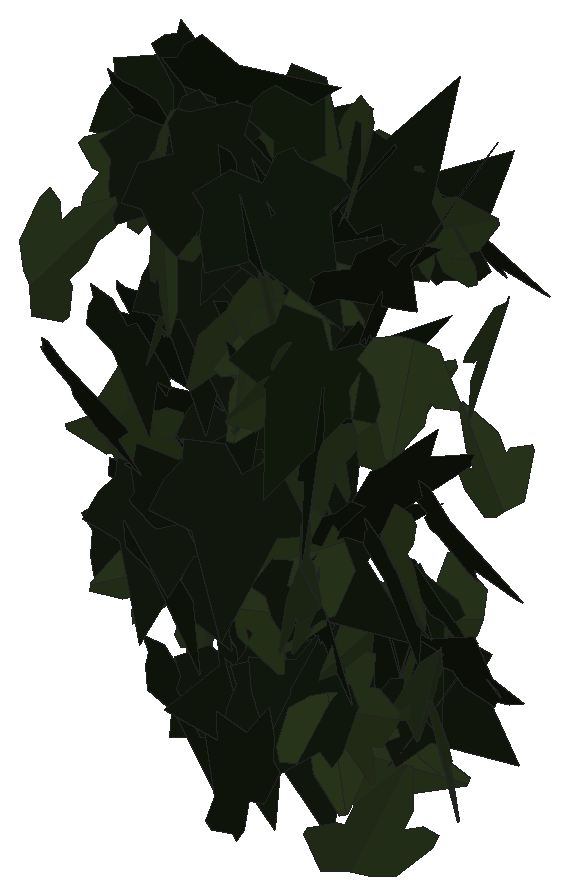
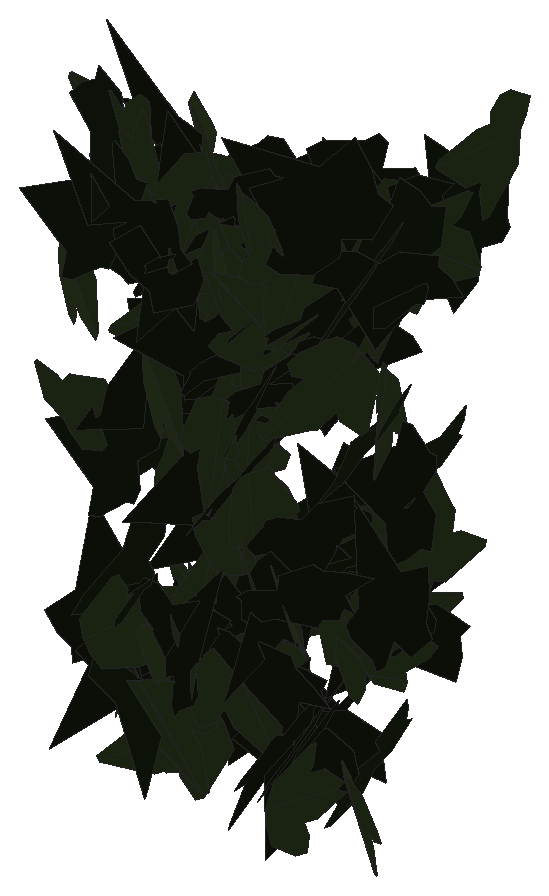
# SketchUp Ruby script. Lengths in inches.
U = 1.inch
M = Sketchup.active_model
def pt(a) = Geom::Point3d.new(a.map { |v| v * U })
def face(e, loops, mat)
  f = e.add_face(loops[0].map { |a| pt(a) })
  loops[1..].each { |l| e.add_face(l.map { |a| pt(a) }).erase! }
  f.material = f.back_material = mat if mat
  f
end
# faces: each face lists its corners as indices into pts; further lists are holes
def faces(e, pts, list, mat = nil) = list.each { |f| face(e, (f[0].is_a?(Array) ? f : [f]).map { |l| l.map { |i| pts[i] } }, mat) }
# xy, xz, yz: faces in a plane at the given z, y or x. An outline is a flat list of corners, or four numbers for a rectangle; further outlines are holes
def ring(l) = l.size == 4 ? [[l[0], l[1]], [l[2], l[1]], [l[2], l[3]], [l[0], l[3]]] : l.each_slice(2).to_a
def flat(e, list, mat, &to3) = list.each { |f| face(e, (f[0].is_a?(Array) ? f : [f]).map { |l| ring(l).map { |u, v| to3.(u, v) } }, mat) }
def xy(e, z, list, mat = nil) = flat(e, list, mat) { |x, y| [x, y, z] }
def xz(e, y, list, mat = nil) = flat(e, list, mat) { |x, z| [x, y, z] }
def yz(e, x, list, mat = nil) = flat(e, list, mat) { |y, z| [x, y, z] }
def lines(e, pts, list) = list.each { |a, b| e.add_line(pt(pts[a]), pt(pts[b])) }
# prism: a flat outline (further loops are holes) pulled along v
def prism(e, loops, v, mat = nil)
  f = face(e, loops, mat); d = Geom::Vector3d.new(v.map { |x| x * U })
  f.pushpull(f.normal.samedirection?(d) ? d.length : -d.length)
end
def box(e, o, s, mat = nil) = prism(e, [[o, [o[0] + s[0], o[1], o[2]], [o[0] + s[0], o[1] + s[1], o[2]], [o[0], o[1] + s[1], o[2]]]], [0, 0, s[2]], mat)
def at(x, y, z, deg = 0) = Geom::Transformation.translation(pt([x, y, z])) * Geom::Transformation.rotation(ORIGIN, Z_AXIS, deg.degrees)
def axes(o, x, y, z) = Geom::Transformation.new([*x, 0, *y, 0, *z, 0, *pt(o).to_a, 1])
def part(name) = M.definitions.add(name)
# library, detail: a bought-in or finely detailed component or shape, given as its bounding box
def library(name, o, s) = part(name).tap { |d| box(d.entities, o, s) }
def detail(e, o, s) = box(e.add_group.entities, o, s)
def put(e, d, t, mat = nil) = e.add_instance(d, t).tap { |i| i.material = mat if mat }
def group(e, t, mat = nil) = e.add_group.tap { |g| g.transformation = t; g.material = mat if mat }.entities
root = M.entities
M.materials.add("efeu1").color = [18, 25, 13]
M.materials.add("efeu2").color = [43, 57, 29]
c1 = part("ivyleaf_9")
p = [[1.54,2.16,1.25],[1.36,2.04,1.19],[-0.21,0.99,0.68],[-0.71,1.11,0.82],[-0.85,0.86,0.67],[-0.8,0.17,0.21],
  [-0.9,-0.01,0.1],[-0.67,-0.16,-0.02],[-0.08,-0.08,-0.05],[-0.03,-0.6,-0.4],[0.65,-0.88,-0.66],[0.83,-0.6,-0.49],
  [1.29,-0.42,-0.43],[1.8125,-0.07,-0.26],[1.21,0.44,0.15]]
faces(c1.entities,p,[[0,1,2,3,4,5,6,7,8,9,10,11,12,13,14]],"efeu1")
c2 = part("ivyleaf_10")
p = [[0,0.5,-0.03],[-0.0625,2.02,-0.43],[-0.19,2.01,-0.46],[-0.54,1.05,-0.29],[-0.52,0.625,-0.18],[-0.83,0.76,-0.28],
  [-1.16,0.64,-0.33],[-1.15,0.33,-0.24],[-0.77,-0.39,0.02],[-0.3,-0.51,0.16],[0.04,-0.48,0.23],[-0.02,2.01,-0.4375],
  [-0.06,2.01,-0.43],[0.04,-0.49,0.23],[0.67,-0.49,0.14],[1.38,0.36,-0.2],[1.375,0.51,-0.24],[0.81,0.65,-0.19],
  [0.62,0.59,-0.15],[0.6,1.09,-0.28],[0.5,1.23,-0.31]]
faces(c2.entities,p,[[0,1,2,3,4,5,6,7,8,9,10],[11,12,0,13,14,15,16,17,18,19,20]],"efeu2")
put(root,c1,axes([530.42,134.07,176.39],[-0.19961,-0.0904,0.83266],[0.51605,-0.68748,0.04907],[0.65969,0.51043,0.21356]))
put(root,c2,axes([531,132.61,177.125],[-0.64831,-0.40875,-0.10208],[-0.0864,-0.05436,0.76641],[-0.41235,0.65404,-0.0001]))
put(root,c1,axes([530.68,132.83,178.89],[0.19641,-0.67069,0.3867],[0.18084,-0.34817,-0.69571],[0.75277,0.25864,0.06623]))
put(root,c1,axes([530.47,133.28,178.82],[0.27402,0.08156,-0.79711],[0.7819,0.15691,0.28484],[0.17513,-0.82816,-0.02453]))
put(root,c1,axes([530.99,133.68,183.2],[-0.40661,-0.63217,-0.4158],[0.23827,0.34104,-0.75152],[0.71816,-0.47108,0.01392]))
put(root,c1,axes([531,134.51,182.88],[-0.01653,-0.63699,0.61836],[0.04917,-0.61818,-0.63549],[0.88641,0.02241,0.04678]))
put(root,c2,axes([531.32,133.98,172.93],[0.60505,-0.49393,0.00823],[0.00635,-0.00524,-0.78106],[0.49396,0.60508,-0.00004]))
put(root,c2,axes([531.55,133.32,175.31],[0.4181,0.66594,0.37045],[-0.20403,-0.30928,0.78627],[0.73422,-0.46517,0.00755]))
put(root,c2,axes([531.55,132,182.63],[-0.16338,-0.46684,0.76473],[0.12017,-0.78174,-0.45155],[0.88787,0.0199,0.20183]))
put(root,c1,axes([530.86,132.93,183],[0.62718,-0.3592,0.49894],[0.43451,-0.24524,-0.72275],[0.43493,0.76298,0.00258]))
put(root,c2,axes([531.77,132.53,180],[0.12734,-0.50966,-0.57524],[-0.12448,0.56171,-0.52522],[0.7584,0.17777,0.01037]))
put(root,c1,axes([531.39,132.53,175.83],[-0.22825,-0.37055,-0.79058],[0.44585,0.65311,-0.43484],[0.7507,-0.50056,0.01788]))
put(root,c1,axes([531.17,132.47,176.17],[0.5641,-0.09914,0.51596],[0.51255,-0.0625,-0.57239],[0.11545,0.76191,0.02018]))
put(root,c2,axes([531.88,132.3,175.09],[-0.11086,0.16475,0.74918],[0.01272,-0.75647,0.16823],[0.76698,0.03636,0.1055]))
put(root,c2,axes([531.8,133.28,175.65],[0.11126,-0.72273,0.55876],[0.13615,-0.54348,-0.73008],[0.90334,0.17093,0.04122]))
put(root,c1,axes([531.56,133.45,179.27],[0.16944,-0.75782,0.35446],[0.12801,-0.33392,-0.77508],[0.82677,0.20701,0.04737]))
put(root,c1,axes([531.83,132.38,176.29],[-0.21329,-0.80961,0.00703],[0.00301,-0.00806,-0.83723],[0.80964,-0.21326,0.00497]))
put(root,c2,axes([531.36,132.37,176.6875],[-0.28979,-0.17322,0.87246],[0.80763,0.33325,0.33442],[-0.37271,0.8568,0.04632]))
put(root,c1,axes([531.54,132.54,175.41],[0.39181,-0.7456,0.3233],[0.13592,-0.29373,-0.84214],[0.80123,0.41443,-0.01524]))
put(root,c2,axes([532.04,132.16,181.375],[-0.12956,0.72713,-0.22495],[0.03146,-0.22288,-0.73854],[-0.76048,-0.1331,0.00777]))
put(root,c2,axes([532.4,132.34,182.13],[-0.6455,-0.4203,0.14551],[-0.1241,-0.07608,-0.77027],[0.42711,-0.65731,-0.00389]))
put(root,c1,axes([532.43,134.57,176.76],[-0.60887,-0.60672,0.12312],[-0.07616,-0.09798,-0.85941],[0.61438,-0.61342,0.01549]))
put(root,c2,axes([532.21,131.89,183.08],[-0.03458,-0.62511,-0.66836],[0.2283,0.6418,-0.61208],[0.8862,-0.18973,0.1316]))
put(root,c1,axes([531.84,132.85,172.75],[0.35181,-0.75777,0.28334],[0.14691,-0.244,-0.83496],[0.79556,0.38016,0.02889]))
put(root,c2,axes([532.09,133.35,180.62],[-0.25827,-0.42652,-0.70004],[0.48268,0.5141,-0.49132],[0.66256,-0.54079,0.08505]))
put(root,c1,axes([532.48,133.9375,181.77],[-0.28546,-0.71382,0.21623],[-0.0505,-0.2125,-0.76816],[0.74414,-0.28825,0.03082]))
put(root,c2,axes([532.52,134.35,172.42],[-0.03744,-0.12912,0.80787],[0.17064,-0.79216,-0.1187],[0.80013,0.1629,0.06312]))
put(root,c2,axes([532.59,128.24,182.75],[0.06432,0.13321,-0.95605],[0.19114,0.93744,0.14348],[0.94618,-0.19843,0.03601]))
put(root,c1,axes([532.29,132,183.48],[-0.00185,-0.65291,-0.69909],[0.18551,0.68557,-0.64078],[0.93841,-0.13681,0.1253]))
put(root,c1,axes([532.48,132.98,180.83],[-0.20242,-0.84849,-0.34592],[0.05894,0.34147,-0.87206],[0.9144,-0.20984,-0.02036]))
put(root,c2,axes([532.72,133.64,182.78],[-0.66465,-0.46754,-0.22362],[0.17552,0.1391,-0.81253],[0.48764,-0.68732,-0.01233]))
put(root,c1,axes([532.6,133.8,177.7],[-0.281,-0.73455,-0.21787],[0.05269,0.21298,-0.78604],[0.76437,-0.28472,-0.0259]))
put(root,c1,axes([532.04,133.58,183.43],[0.16917,-0.274,0.85823],[0.83818,-0.27226,-0.25214],[0.33028,0.83129,0.20029]))
put(root,c1,axes([532.4375,132.21,176.26],[-0.37873,-0.09053,0.74585],[0.73748,-0.2044,0.34967],[0.14357,0.81114,0.17136]))
put(root,c1,axes([532.6,134.1,173.34],[0.05998,-0.71944,0.45891],[0.01209,-0.45928,-0.7216],[0.85326,0.05708,-0.02204]))
put(root,c1,axes([533.11,132.85,172.95],[0.35814,0.70014,0.06005],[0.0263,0.054,-0.78642],[-0.70221,0.35911,0.00118]))
put(root,c1,axes([533.2,133.32,176.3],[0.0602,-0.04516,-0.89711],[-0.55577,0.70448,-0.07276],[0.70566,0.55869,0.01923]))
put(root,c1,axes([532.87,134.03,173.48],[0.35128,-0.64102,-0.32987],[-0.161,0.28793,-0.73096],[0.70271,0.38641,-0.00257]))
put(root,c2,axes([533.09,133.74,176.32],[0.45669,-0.62733,0.2177],[0.12812,-0.17601,-0.77596],[0.65155,0.47432,-0.00001]))
put(root,c1,axes([532.8125,131.52,183.46],[0.22851,-0.12055,-0.89764],[0.07424,0.92515,-0.10535],[0.90265,-0.04557,0.23591]))
put(root,c1,axes([533.21,133.05,172.61],[0.29325,-0.67869,-0.44546],[0.22228,-0.3884,0.73809],[-0.78079,-0.36548,0.04282]))
put(root,c1,axes([533.32,134.22,175.04],[-0.73437,-0.25317,-0.39205],[0.36152,0.15365,-0.7764],[0.29513,-0.81817,-0.02449]))
put(root,c1,axes([532.67,132.43,177.01],[0.631,-0.48552,0.42101],[0.33166,-0.25935,-0.79617],[0.55044,0.71285,-0.00292]))
put(root,c1,axes([533.03,132.71,173.3125],[-0.39956,-0.4007,-0.6967],[0.57097,0.40606,-0.561],[0.56564,-0.69294,0.07414]))
put(root,c2,axes([533.17,133.95,181.1875],[-0.35472,-0.52179,0.45423],[0.23726,0.38775,0.6307],[-0.64985,0.42639,-0.01768]))
put(root,c1,axes([533.4,133.86,180.16],[-0.33223,-0.66755,0.21984],[-0.08734,-0.20207,-0.74557],[0.69737,-0.34334,0.01135]))
put(root,c2,axes([533.31,133.63,176.03],[-0.04436,-0.10074,0.81796],[0.2995,-0.7651,-0.07798],[0.76779,0.29264,0.07768]))
put(root,c2,axes([533.57,133.94,177.87],[0.04198,-0.81763,-0.16606],[-0.02181,0.16514,-0.81861],[0.83404,0.04547,-0.01304]))
put(root,c1,axes([533.14,133.49,182.71],[-0.02434,-0.4959,0.68379],[0.27744,-0.65081,-0.46211],[0.79781,0.21119,0.18156]))
put(root,c1,axes([533.49,133.15,176.8],[-0.63519,-0.44885,-0.39356],[0.31931,0.23008,-0.77777],[0.50438,-0.71092,-0.00324]))
put(root,c1,axes([533.19,132.8,179.78],[0.4901,-0.63824,0.10982],[0.05657,-0.095,-0.80461],[0.64515,0.49319,-0.01287]))
put(root,c2,axes([533.62,131.9375,180.47],[-0.1813,-0.7313,-0.51435],[0.2213,0.47178,-0.74879],[0.86625,-0.27358,0.08364]))
put(root,c1,axes([533.19,132.08,182.95],[0.13828,-0.14266,-0.76129],[0.77454,0.02489,0.13602],[-0.00058,-0.77334,0.14481]))
put(root,c2,axes([534.04,133.88,174.41],[-0.45477,-0.66197,0.34515],[-0.17495,-0.2984,-0.80281],[0.72576,-0.48673,0.02276]))
put(root,c1,axes([533.11,128.39,180.59],[0.73885,-0.08875,-0.62221],[0.619,-0.06371,0.74411],[-0.10894,-0.96384,0.00811]))
put(root,c1,axes([533.76,133.95,179.29],[-0.22343,-0.26499,0.81358],[-0.14365,-0.81731,-0.30565],[0.8435,-0.20938,0.16345]))
put(root,c2,axes([533.67,133.93,183.52],[0.71251,-0.28692,0.18707],[0.17754,-0.05987,-0.76804],[0.29291,0.73422,0.01048]))
put(root,c2,axes([533.92,132.71,180.25],[0.08535,-0.6148,0.53097],[0.16972,-0.50862,-0.61619],[0.79442,0.17471,0.0746]))
put(root,c1,axes([534.06,133.9,183.7],[-0.51178,-0.59635,-0.02477],[0.01964,0.01579,-0.78583],[0.59654,-0.51213,0.00462]))
put(root,c1,axes([533.89,134.33,180.81],[-0.14109,-0.77425,0.21004],[-0.02941,-0.20813,-0.78696],[0.80169,-0.1439,0.0081]))
put(root,c2,axes([534.15,132.36,179.83],[0.61454,0.40623,-0.30525],[-0.25801,-0.16322,-0.73665],[-0.43776,0.66648,0.00565]))
put(root,c1,axes([534.7,130.93,172.38],[-0.12688,0.29665,0.76444],[-0.42858,0.63548,-0.31774],[-0.69907,-0.44344,0.05606]))
put(root,c2,axes([534.25,132.78,180.09],[0.03506,-0.54942,0.77103],[0.16579,-0.75608,-0.54631],[0.93213,0.15514,0.06816]))
put(root,c2,axes([534.3125,133.73,182.46],[0.23506,-0.75198,0.05685],[0.02459,-0.05187,-0.78783],[0.75373,0.23621,0.00798]))
put(root,c2,axes([534.47,133.86,179.02],[-0.69272,0.29849,0.21379],[-0.19844,0.07971,-0.75428],[-0.30891,-0.72056,0.00512]))
put(root,c1,axes([533.95,133.9,178.11],[0.21486,-0.80881,0.04294],[0.01374,-0.04078,-0.83686],[0.80984,0.21528,0.0028]))
put(root,c2,axes([534.23,133.4375,176.46],[-0.76964,-0.15658,0.27459],[0.27956,0.00012,0.78365],[-0.14752,0.81716,0.0525]))
put(root,c2,axes([533.86,132.22,175.05],[0.14103,-0.11162,-0.76977],[0.75553,-0.16626,0.16253],[-0.18485,-0.76471,0.07702]))
put(root,c2,axes([534.34,131.96,181.19],[-0.39755,0.59175,-0.36069],[0.18463,-0.31035,-0.71267],[-0.66796,-0.43797,0.01768]))
put(root,c1,axes([534.38,132.6,173.61],[-0.43753,-0.4306,-0.66005],[0.4522,0.48113,-0.61363],[0.64544,-0.62898,-0.01753]))
put(root,c2,axes([534.1875,133.9,182.43],[0.60144,-0.09468,0.57021],[0.56644,-0.06728,-0.60864],[0.11507,0.82604,0.01579]))
put(root,c1,axes([534.36,131.84,183.25],[-0.12528,-0.55746,-0.72596],[0.21273,0.69493,-0.57034],[0.89024,-0.2445,0.03413]))
put(root,c1,axes([534.9,132.6,173.0625],[-0.66939,-0.04287,0.56254],[0.56242,0.01804,0.67062],[-0.04444,0.87419,0.01375]))
put(root,c1,axes([534.34,132.89,175.7],[0.0779,0.00901,-0.93338],[0.931,-0.06824,0.07704],[-0.06726,-0.93414,-0.01463]))
put(root,c1,axes([535.25,133.95,173.95],[0.27603,-0.53448,0.66931],[-0.22882,0.63163,0.59876],[-0.8254,-0.35384,0.05784]))
put(root,c2,axes([534.98,133.31,183.34],[-0.48615,-0.59628,-0.33744],[0.22356,0.25305,-0.76925],[0.64764,-0.53495,0.01224]))
put(root,c1,axes([534.91,130.49,178.5625],[-0.25399,-0.87749,-0.09441],[0.03801,0.08727,-0.91342],[0.88173,-0.25653,0.01218]))
put(root,c2,axes([535.54,131.86,176.93],[0.44424,-0.00115,-0.6705],[-0.6622,0.12545,-0.43895],[0.10521,0.79447,0.06834]))
put(root,c2,axes([535.17,131.97,178.55],[-0.31059,-0.84992,-0.15469],[0.05099,0.14606,-0.90489],[0.86237,-0.31474,-0.0022]))
put(root,c1,axes([535.47,132.35,174.08],[-0.88211,0.19549,-0.12307],[0.11986,-0.02797,-0.90351],[-0.19748,-0.89022,0.00136]))
put(root,c2,axes([535.2,131.45,180.11],[-0.0504,0.01155,-0.83258],[-0.1594,-0.81881,-0.00171],[-0.81726,0.15899,0.05167]))
put(root,c1,axes([535.08,133.83,182.11],[-0.28704,-0.84979,0.06163],[-0.01517,-0.05993,-0.89694],[0.85188,-0.2874,0.00479]))
put(root,c2,axes([535.31,132.14,176.12],[-0.00958,-0.59114,-0.69461],[0.03049,0.69405,-0.59109],[0.91159,-0.02942,0.01247]))
put(root,c1,axes([535,133.47,181.74],[0.65269,0.59618,0.38423],[-0.29185,-0.25016,0.88392],[0.64644,-0.71488,0.01112]))
put(root,c2,axes([535.43,132.99,184],[0.61549,-0.75122,-0.17987],[-0.1117,0.14101,-0.97116],[0.76433,0.62554,0.00291]))
put(root,c1,axes([534.68,133.3,174.05],[0.20188,-0.06845,0.80448],[0.74141,-0.3126,-0.21265],[0.31966,0.76826,-0.01485]))
put(root,c2,axes([535.2,132.08,181.375],[0.19744,0.68911,0.3655],[0.10552,0.34997,-0.71682],[-0.77287,0.22382,-0.0045]))
put(root,c2,axes([535.68,133.94,173.2],[0.82797,-0.10908,-0.34609],[-0.34322,0.04451,-0.83512],[0.11781,0.89629,-0.00065]))
put(root,c2,axes([535.41,133.39,174.8],[-0.00667,-0.06635,0.80524],[0.25916,-0.7629,-0.06072],[0.76528,0.25778,0.02758]))
put(root,c1,axes([535.13,131.99,176.42],[0.00887,-0.15204,-0.78653],[0.27612,0.73896,-0.13973],[0.752,-0.26954,0.06059]))
put(root,c1,axes([535.5,132.1,176.87],[0.30763,0.38852,0.64373],[0.38916,0.51285,-0.4955],[-0.64335,0.496,0.00809]))
put(root,c1,axes([536.03,132.98,181.58],[-0.22018,0.18806,-0.79851],[-0.60099,0.52578,0.28954],[0.55839,0.64005,-0.00323]))
put(root,c2,axes([535.5,132.1,173.6],[0.66279,0.41634,0.17648],[0.14516,0.10067,-0.78267],[-0.42827,0.67845,0.00784]))
put(root,c1,axes([535.39,133.87,175.08],[-0.3185,-0.40667,-0.6645],[0.47328,0.46923,-0.51401],[0.61882,-0.56818,0.05111]))
put(root,c1,axes([535.53,132.32,179.625],[0.12239,0.16249,0.78214],[0.54754,0.5591,-0.20183],[-0.58167,0.56047,-0.02542]))
put(root,c2,axes([535.35,133.24,172.4375],[-0.26863,-0.16514,-0.80042],[0.72795,0.33466,-0.31335],[0.37152,-0.77513,0.03523]))
put(root,c1,axes([535.91,131.5,180.8125],[-0.57367,-0.65305,-0.05444],[0.03488,0.04182,-0.86924],[0.65439,-0.57473,-0.00139]))
put(root,c1,axes([536.36,133.64,173.33],[-0.18096,0.76154,0.32734],[-0.07968,0.31752,-0.78274],[-0.82507,-0.19769,0.0038]))
put(root,c2,axes([536.21,134.58,174.65],[0.04545,0.23688,0.7628],[-0.13777,-0.75026,0.24119],[0.78676,-0.14506,-0.00183]))
put(root,c2,axes([535.88,133.625,173.88],[0.45252,-0.70845,-0.29478],[0.15559,-0.2504,0.84063],[-0.75139,-0.47851,-0.00346]))
put(root,c2,axes([536.27,130.33,177.39],[0.24478,-0.6296,-0.63071],[-0.06346,0.64009,-0.6636],[0.88891,0.21907,0.1263]))
put(root,c2,axes([536.13,133.39,179.28],[0.36912,-0.7897,0.23296],[0.10494,-0.20809,-0.87168],[0.81663,0.38369,0.00672]))
put(root,c1,axes([536.21,131.87,182.39],[0.42475,0.68591,0.09505],[0.05079,0.08035,-0.80678],[-0.6906,0.42777,-0.00087]))
put(root,c1,axes([535.98,131.13,179.82],[-0.29748,-0.01021,-0.78546],[0.75816,-0.22351,-0.28423],[-0.20555,-0.80962,0.08837]))
put(root,c1,axes([535.91,134.09,181.9],[-0.31728,0.19408,0.80129],[0.69328,-0.40187,0.37185],[0.4462,0.76239,-0.00797]))
put(root,c2,axes([536.3125,132,171.4],[-0.45345,-0.75182,0.26332],[0.13408,0.22664,0.87798],[-0.78524,0.47286,-0.00214]))
put(root,c2,axes([535.93,132.19,173.875],[0.22242,-0.21006,-0.8027],[0.63531,-0.49143,0.30464],[-0.53371,-0.67253,0.02811]))
put(root,c1,axes([536.26,133.6,173.88],[0.06906,-0.29872,-0.75237],[-0.05302,0.75181,-0.30337],[0.80777,0.07489,0.04441]))
put(root,c1,axes([536.29,132.55,183.11],[-0.56653,0.52634,0.60272],[0.44363,-0.408,0.77329],[0.66595,0.71955,-0.0024]))
put(root,c1,axes([536.08,133.76,175.7],[0.64137,-0.47632,0.05544],[0.04731,-0.02929,-0.79888],[0.47719,0.6431,0.00468]))
put(root,c2,axes([536.68,133.31,174.48],[0.10949,-0.77654,-0.049],[-0.00657,0.04856,-0.78422],[0.77806,0.10969,0.00027]))
put(root,c2,axes([536.62,131.86,179.73],[0.09337,0.07205,-0.92569],[0.30249,0.87724,0.09879],[0.87783,-0.30995,0.06442]))
put(root,c2,axes([536.28,133.45,182.87],[-0.04848,0.01227,0.86142],[0.84459,-0.16948,0.04995],[0.16991,0.84597,-0.00249]))
put(root,c1,axes([536.78,131.6,178.32],[0.34546,0.49988,0.72766],[0.36563,0.63021,-0.60652],[-0.80355,0.50166,0.03685]))
put(root,c2,axes([536.84,133.26,173.45],[-0.43725,0.57651,-0.30835],[0.19209,-0.2413,-0.72354],[-0.62493,-0.47754,-0.00665]))
put(root,c1,axes([537.35,132.74,183.32],[0.01578,0.65304,0.55848],[-0.015,0.5587,-0.65288],[-0.85915,0.00224,0.02166]))
put(root,c1,axes([536.47,134.23,182.31],[0.43092,-0.42356,0.57102],[0.48472,-0.31345,-0.5983],[0.52012,0.64305,0.08448]))
put(root,c1,axes([536.79,133.76,174.24],[0.75962,-0.06089,-0.07264],[0.07258,-0.00362,0.76205],[-0.06096,-0.76307,0.00218]))
put(root,c2,axes([537.15,132.05,180.85],[0.81326,0.10424,-0.01068],[-0.0106,-0.0013,-0.81991],[-0.10424,0.81333,0.00006]))
put(root,c2,axes([536.83,132.17,177.15],[-0.11501,0.15651,-0.96489],[0.62233,-0.73749,-0.1938],[-0.7538,-0.63274,-0.01278]))
put(root,c1,axes([536.69,133.29,177.3],[0.48061,-0.42717,0.63079],[0.46506,-0.42622,-0.64297],[0.6034,0.66874,-0.00687]))
put(root,c2,axes([537.74,133.72,177.99],[0.58246,0.01244,0.47439],[-0.47425,-0.01166,0.58259],[0.017,-0.75112,-0.00119]))
put(root,c1,axes([537.11,131.8,177.06],[0.23406,-0.56495,0.55341],[0.21248,-0.51099,-0.61151],[0.76176,0.31612,0.00053]))
put(root,c2,axes([537.13,132.95,182.95],[-0.46445,0.00375,0.71478],[0.71465,0.01936,0.46426],[-0.01419,0.8522,-0.01369]))
put(root,c2,axes([537.64,133.79,181.03],[0.29466,-0.72997,0.22228],[0.09751,-0.20031,-0.78706],[0.75681,0.31002,0.01486]))
